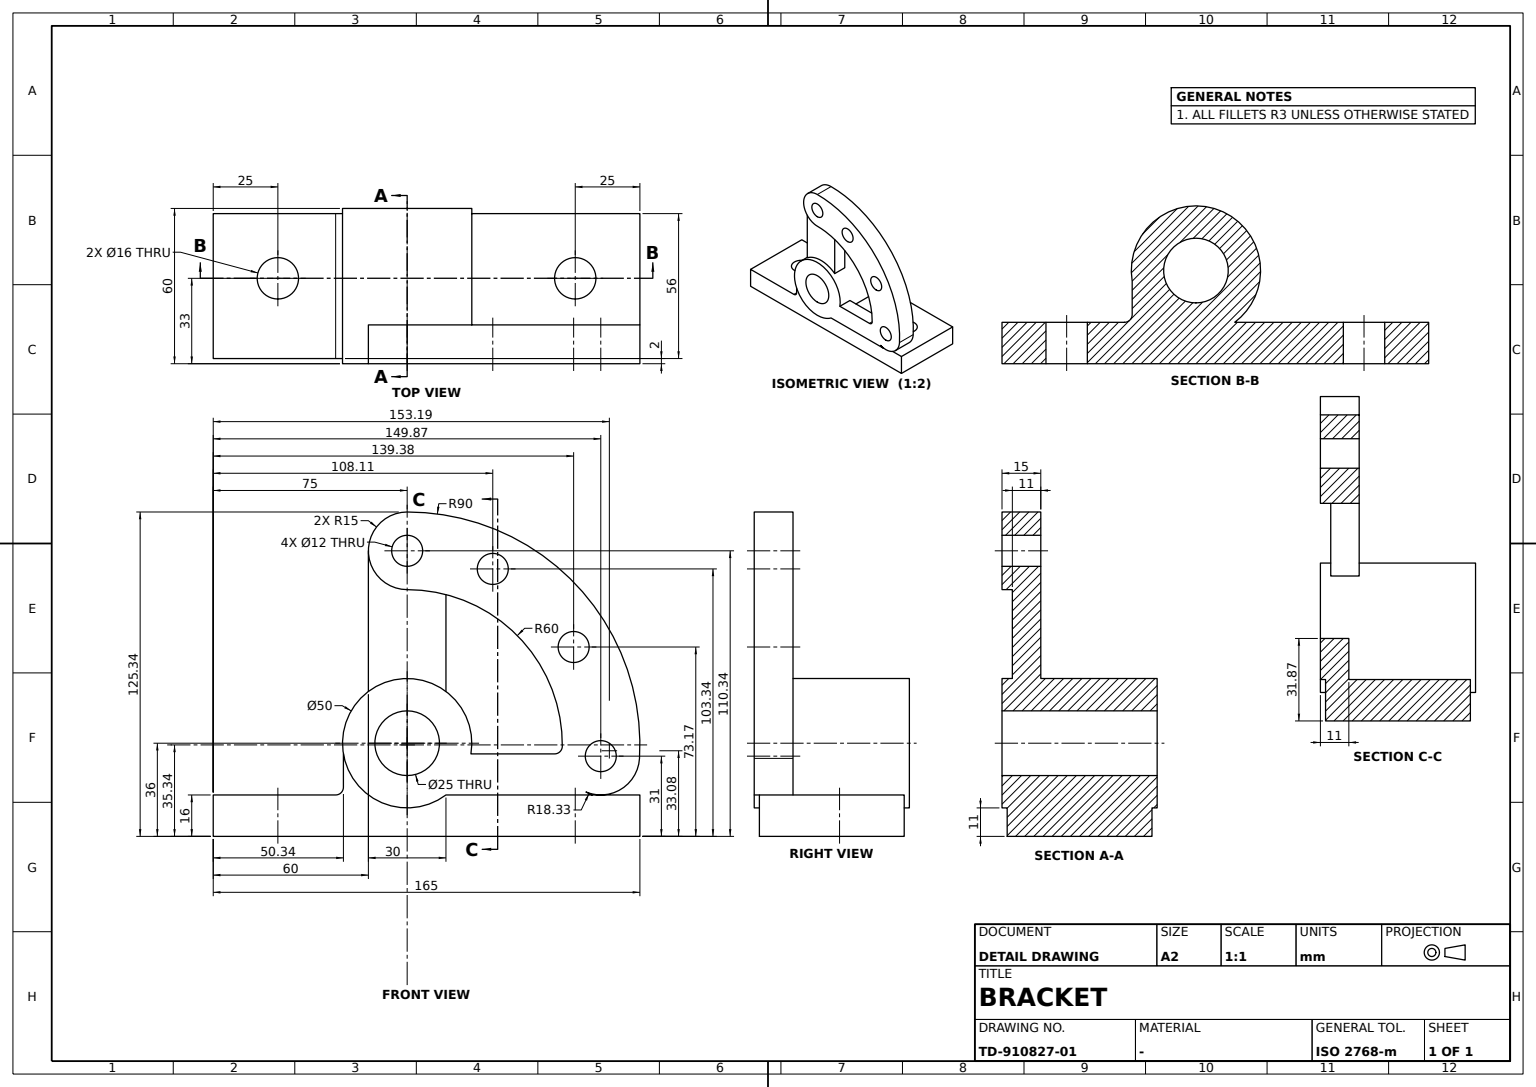
ISO-10303-21;
HEADER;
FILE_DESCRIPTION((''),'2;1');
FILE_NAME('','',(''),(''),'','','');
FILE_SCHEMA(('AUTOMOTIVE_DESIGN'));
ENDSEC;
DATA;
#1=APPLICATION_CONTEXT('');
#2=PRODUCT_CONTEXT('',#1,'mechanical');
#3=PRODUCT('','','',(#2));
#4=PRODUCT_DEFINITION_FORMATION('','',#3);
#5=PRODUCT_DEFINITION_CONTEXT('',#1,'design');
#6=PRODUCT_DEFINITION('','',#4,#5);
#7=PRODUCT_DEFINITION_SHAPE('','',#6);
#8=(LENGTH_UNIT()NAMED_UNIT(*)SI_UNIT(.MILLI.,.METRE.));
#9=(NAMED_UNIT(*)PLANE_ANGLE_UNIT()SI_UNIT($,.RADIAN.));
#10=(NAMED_UNIT(*)SI_UNIT($,.STERADIAN.)SOLID_ANGLE_UNIT());
#11=UNCERTAINTY_MEASURE_WITH_UNIT(LENGTH_MEASURE(0.005),#8,'distance_accuracy_value','');
#12=(GEOMETRIC_REPRESENTATION_CONTEXT(3)GLOBAL_UNCERTAINTY_ASSIGNED_CONTEXT((#11))GLOBAL_UNIT_ASSIGNED_CONTEXT((#8,#9,#10))REPRESENTATION_CONTEXT('',''));
#13=CARTESIAN_POINT('',(15.,0.,104.3383901));
#14=VERTEX_POINT('',#13);
#15=CARTESIAN_POINT('',(15.,0.,110.3383901));
#16=DIRECTION('',(1.,0.,0.));
#17=DIRECTION('',(0.,0.,-1.));
#18=AXIS2_PLACEMENT_3D('',#15,#16,#17);
#19=CIRCLE('',#18,6.);
#20=EDGE_CURVE('',#14,#14,#19,.T.);
#21=ORIENTED_EDGE('',*,*,#20,.T.);
#22=EDGE_LOOP('',(#21));
#23=FACE_BOUND('',#22,.T.);
#24=CARTESIAN_POINT('',(15.,64.37893431,67.16919505));
#25=VERTEX_POINT('',#24);
#26=CARTESIAN_POINT('',(15.,64.37893431,73.16919505));
#27=AXIS2_PLACEMENT_3D('',#26,#16,#17);
#28=CIRCLE('',#27,6.);
#29=EDGE_CURVE('',#25,#25,#28,.T.);
#30=ORIENTED_EDGE('',*,*,#29,.T.);
#31=EDGE_LOOP('',(#30));
#32=FACE_BOUND('',#31,.T.);
#33=CARTESIAN_POINT('',(15.,74.87441734,25.));
#34=VERTEX_POINT('',#33);
#35=CARTESIAN_POINT('',(15.,74.87441734,31.));
#36=AXIS2_PLACEMENT_3D('',#35,#16,#17);
#37=CIRCLE('',#36,6.);
#38=EDGE_CURVE('',#34,#34,#37,.T.);
#39=ORIENTED_EDGE('',*,*,#38,.T.);
#40=EDGE_LOOP('',(#39));
#41=FACE_BOUND('',#40,.T.);
#42=CARTESIAN_POINT('',(15.,33.10708165,97.34314751));
#43=VERTEX_POINT('',#42);
#44=CARTESIAN_POINT('',(15.,33.10708165,103.34314751));
#45=AXIS2_PLACEMENT_3D('',#44,#16,#17);
#46=CIRCLE('',#45,6.);
#47=EDGE_CURVE('',#43,#43,#46,.T.);
#48=ORIENTED_EDGE('',*,*,#47,.T.);
#49=EDGE_LOOP('',(#48));
#50=FACE_BOUND('',#49,.T.);
#51=CARTESIAN_POINT('',(15.,-15.,110.3383901));
#52=VERTEX_POINT('',#51);
#53=CARTESIAN_POINT('',(15.,-15.,56.));
#54=VERTEX_POINT('',#53);
#55=CARTESIAN_POINT('',(15.,-15.,0.));
#56=VECTOR('',#17,1000.);
#57=LINE('',#55,#56);
#58=EDGE_CURVE('',#52,#54,#57,.T.);
#59=ORIENTED_EDGE('',*,*,#58,.F.);
#60=CARTESIAN_POINT('',(15.,0.,125.3383901));
#61=VERTEX_POINT('',#60);
#62=CIRCLE('',#18,15.);
#63=EDGE_CURVE('',#61,#52,#62,.T.);
#64=ORIENTED_EDGE('',*,*,#63,.F.);
#65=CARTESIAN_POINT('',(15.,89.8493008,30.13232198));
#66=VERTEX_POINT('',#65);
#67=CARTESIAN_POINT('',(15.,0.,35.3383901));
#68=AXIS2_PLACEMENT_3D('',#67,#16,#17);
#69=CIRCLE('',#68,90.);
#70=EDGE_CURVE('',#66,#61,#69,.T.);
#71=ORIENTED_EDGE('',*,*,#70,.F.);
#72=CARTESIAN_POINT('',(15.,59.89953387,31.86767802));
#73=VERTEX_POINT('',#72);
#74=CIRCLE('',#36,15.);
#75=EDGE_CURVE('',#73,#66,#74,.T.);
#76=ORIENTED_EDGE('',*,*,#75,.F.);
#77=CARTESIAN_POINT('',(15.,15.,93.4331403));
#78=VERTEX_POINT('',#77);
#79=CIRCLE('',#68,60.);
#80=EDGE_CURVE('',#73,#78,#79,.T.);
#81=ORIENTED_EDGE('',*,*,#80,.T.);
#82=CARTESIAN_POINT('',(15.,15.,56.));
#83=VERTEX_POINT('',#82);
#84=CARTESIAN_POINT('',(15.,15.,0.));
#85=LINE('',#84,#56);
#86=EDGE_CURVE('',#78,#83,#85,.T.);
#87=ORIENTED_EDGE('',*,*,#86,.T.);
#88=CARTESIAN_POINT('',(15.,0.,36.));
#89=AXIS2_PLACEMENT_3D('',#88,#16,#17);
#90=CIRCLE('',#89,25.);
#91=EDGE_CURVE('',#54,#83,#90,.F.);
#92=ORIENTED_EDGE('',*,*,#91,.F.);
#93=EDGE_LOOP('',(#59,#64,#71,#76,#81,#87,#92));
#94=FACE_BOUND('',#93,.T.);
#95=CARTESIAN_POINT('',(15.,0.,0.));
#96=DIRECTION('',(0.,1.,0.));
#97=AXIS2_PLACEMENT_3D('',#95,#16,#96);
#98=PLANE('',#97);
#99=ADVANCED_FACE('',(#23,#32,#41,#50,#94),#98,.F.);
#100=CARTESIAN_POINT('',(28.,-27.65611314,16.));
#101=VERTEX_POINT('',#100);
#102=CARTESIAN_POINT('',(28.,-75.,16.));
#103=VERTEX_POINT('',#102);
#104=CARTESIAN_POINT('',(28.,0.,16.));
#105=DIRECTION('',(0.,-1.,0.));
#106=VECTOR('',#105,1000.);
#107=LINE('',#104,#106);
#108=EDGE_CURVE('',#101,#103,#107,.T.);
#109=ORIENTED_EDGE('',*,*,#108,.T.);
#110=CARTESIAN_POINT('',(28.,-75.,0.));
#111=VERTEX_POINT('',#110);
#112=LINE('',#110,#56);
#113=EDGE_CURVE('',#103,#111,#112,.T.);
#114=ORIENTED_EDGE('',*,*,#113,.T.);
#115=CARTESIAN_POINT('',(28.,90.,0.));
#116=VERTEX_POINT('',#115);
#117=CARTESIAN_POINT('',(28.,0.,0.));
#118=VECTOR('',#96,1000.);
#119=LINE('',#117,#118);
#120=EDGE_CURVE('',#111,#116,#119,.T.);
#121=ORIENTED_EDGE('',*,*,#120,.T.);
#122=CARTESIAN_POINT('',(28.,90.,16.));
#123=VERTEX_POINT('',#122);
#124=DIRECTION('',(0.,0.,1.));
#125=VECTOR('',#124,1000.);
#126=LINE('',#115,#125);
#127=EDGE_CURVE('',#116,#123,#126,.T.);
#128=ORIENTED_EDGE('',*,*,#127,.T.);
#129=CARTESIAN_POINT('',(28.,71.53640747,16.));
#130=VERTEX_POINT('',#129);
#131=EDGE_CURVE('',#123,#130,#107,.T.);
#132=ORIENTED_EDGE('',*,*,#131,.T.);
#133=CARTESIAN_POINT('',(28.,15.,16.));
#134=VERTEX_POINT('',#133);
#135=EDGE_CURVE('',#130,#134,#107,.T.);
#136=ORIENTED_EDGE('',*,*,#135,.T.);
#137=CARTESIAN_POINT('',(28.,-24.65611314,31.86767802));
#138=VERTEX_POINT('',#137);
#139=CARTESIAN_POINT('',(28.,0.,36.));
#140=AXIS2_PLACEMENT_3D('',#139,#16,#17);
#141=CIRCLE('',#140,25.);
#142=EDGE_CURVE('',#138,#134,#141,.T.);
#143=ORIENTED_EDGE('',*,*,#142,.F.);
#144=CARTESIAN_POINT('',(28.,-24.65611314,19.));
#145=VERTEX_POINT('',#144);
#146=LINE('',#137,#56);
#147=EDGE_CURVE('',#138,#145,#146,.T.);
#148=ORIENTED_EDGE('',*,*,#147,.T.);
#149=CARTESIAN_POINT('',(28.,-27.65611314,19.));
#150=AXIS2_PLACEMENT_3D('',#149,#16,#17);
#151=CIRCLE('',#150,3.);
#152=EDGE_CURVE('',#101,#145,#151,.T.);
#153=ORIENTED_EDGE('',*,*,#152,.F.);
#154=EDGE_LOOP('',(#109,#114,#121,#128,#132,#136,#143,#148,#153));
#155=FACE_BOUND('',#154,.T.);
#156=AXIS2_PLACEMENT_3D('',#117,#16,#96);
#157=PLANE('',#156);
#158=ADVANCED_FACE('',(#155),#157,.T.);
#159=CARTESIAN_POINT('',(-11.,-50.,0.));
#160=VERTEX_POINT('',#159);
#161=CARTESIAN_POINT('',(-3.,-50.,0.));
#162=DIRECTION('',(-1.,0.,0.));
#163=AXIS2_PLACEMENT_3D('',#161,#17,#162);
#164=CIRCLE('',#163,8.);
#165=EDGE_CURVE('',#160,#160,#164,.T.);
#166=ORIENTED_EDGE('',*,*,#165,.T.);
#167=EDGE_LOOP('',(#166));
#168=FACE_BOUND('',#167,.T.);
#169=CARTESIAN_POINT('',(5.,-50.,16.));
#170=VERTEX_POINT('',#169);
#171=CARTESIAN_POINT('',(-3.,-50.,16.));
#172=AXIS2_PLACEMENT_3D('',#171,#124,#16);
#173=CIRCLE('',#172,8.);
#174=EDGE_CURVE('',#170,#170,#173,.T.);
#175=ORIENTED_EDGE('',*,*,#174,.T.);
#176=EDGE_LOOP('',(#175));
#177=FACE_BOUND('',#176,.T.);
#178=CARTESIAN_POINT('',(-3.,-50.,7.34));
#179=AXIS2_PLACEMENT_3D('',#178,#124,#16);
#180=CYLINDRICAL_SURFACE('',#179,8.);
#181=ADVANCED_FACE('',(#168,#177),#180,.F.);
#182=CARTESIAN_POINT('',(-28.,-27.65611314,16.));
#183=VERTEX_POINT('',#182);
#184=CARTESIAN_POINT('',(-28.,-75.,16.));
#185=VERTEX_POINT('',#184);
#186=CARTESIAN_POINT('',(-28.,0.,16.));
#187=LINE('',#186,#106);
#188=EDGE_CURVE('',#183,#185,#187,.T.);
#189=ORIENTED_EDGE('',*,*,#188,.F.);
#190=CARTESIAN_POINT('',(-28.,-24.65611314,19.));
#191=VERTEX_POINT('',#190);
#192=CARTESIAN_POINT('',(-28.,-27.65611314,19.));
#193=AXIS2_PLACEMENT_3D('',#192,#16,#17);
#194=CIRCLE('',#193,3.);
#195=EDGE_CURVE('',#183,#191,#194,.T.);
#196=ORIENTED_EDGE('',*,*,#195,.T.);
#197=CARTESIAN_POINT('',(-28.,-24.65611314,31.86767802));
#198=VERTEX_POINT('',#197);
#199=LINE('',#197,#56);
#200=EDGE_CURVE('',#198,#191,#199,.T.);
#201=ORIENTED_EDGE('',*,*,#200,.F.);
#202=CARTESIAN_POINT('',(-28.,15.,16.));
#203=VERTEX_POINT('',#202);
#204=CARTESIAN_POINT('',(-28.,0.,36.));
#205=AXIS2_PLACEMENT_3D('',#204,#16,#17);
#206=CIRCLE('',#205,25.);
#207=EDGE_CURVE('',#198,#203,#206,.T.);
#208=ORIENTED_EDGE('',*,*,#207,.T.);
#209=CARTESIAN_POINT('',(-28.,90.,16.));
#210=VERTEX_POINT('',#209);
#211=EDGE_CURVE('',#210,#203,#187,.T.);
#212=ORIENTED_EDGE('',*,*,#211,.F.);
#213=CARTESIAN_POINT('',(-28.,90.,0.));
#214=VERTEX_POINT('',#213);
#215=LINE('',#213,#125);
#216=EDGE_CURVE('',#214,#210,#215,.T.);
#217=ORIENTED_EDGE('',*,*,#216,.F.);
#218=CARTESIAN_POINT('',(-28.,-75.,0.));
#219=VERTEX_POINT('',#218);
#220=CARTESIAN_POINT('',(-28.,0.,0.));
#221=LINE('',#220,#118);
#222=EDGE_CURVE('',#219,#214,#221,.T.);
#223=ORIENTED_EDGE('',*,*,#222,.F.);
#224=LINE('',#218,#56);
#225=EDGE_CURVE('',#185,#219,#224,.T.);
#226=ORIENTED_EDGE('',*,*,#225,.F.);
#227=EDGE_LOOP('',(#189,#196,#201,#208,#212,#217,#223,#226));
#228=FACE_BOUND('',#227,.T.);
#229=AXIS2_PLACEMENT_3D('',#220,#16,#96);
#230=PLANE('',#229);
#231=ADVANCED_FACE('',(#228),#230,.F.);
#232=ORIENTED_EDGE('',*,*,#200,.T.);
#233=CARTESIAN_POINT('',(0.,-24.65611314,19.));
#234=VECTOR('',#16,1000.);
#235=LINE('',#233,#234);
#236=EDGE_CURVE('',#191,#145,#235,.T.);
#237=ORIENTED_EDGE('',*,*,#236,.T.);
#238=ORIENTED_EDGE('',*,*,#147,.F.);
#239=LINE('',#137,#234);
#240=EDGE_CURVE('',#138,#198,#239,.F.);
#241=ORIENTED_EDGE('',*,*,#240,.T.);
#242=EDGE_LOOP('',(#232,#237,#238,#241));
#243=FACE_BOUND('',#242,.T.);
#244=AXIS2_PLACEMENT_3D('',#137,#96,#17);
#245=PLANE('',#244);
#246=ADVANCED_FACE('',(#243),#245,.F.);
#247=CARTESIAN_POINT('',(30.,33.10708165,97.34314751));
#248=VERTEX_POINT('',#247);
#249=CARTESIAN_POINT('',(30.,33.10708165,103.34314751));
#250=AXIS2_PLACEMENT_3D('',#249,#16,#17);
#251=CIRCLE('',#250,6.);
#252=EDGE_CURVE('',#248,#248,#251,.T.);
#253=ORIENTED_EDGE('',*,*,#252,.T.);
#254=EDGE_LOOP('',(#253));
#255=FACE_BOUND('',#254,.T.);
#256=ORIENTED_EDGE('',*,*,#47,.F.);
#257=EDGE_LOOP('',(#256));
#258=FACE_BOUND('',#257,.T.);
#259=CARTESIAN_POINT('',(-0.66,33.10708165,103.34314751));
#260=AXIS2_PLACEMENT_3D('',#259,#16,#96);
#261=CYLINDRICAL_SURFACE('',#260,6.);
#262=ADVANCED_FACE('',(#255,#258),#261,.F.);
#263=CARTESIAN_POINT('',(30.,0.,104.3383901));
#264=VERTEX_POINT('',#263);
#265=CARTESIAN_POINT('',(30.,0.,110.3383901));
#266=AXIS2_PLACEMENT_3D('',#265,#16,#17);
#267=CIRCLE('',#266,6.);
#268=EDGE_CURVE('',#264,#264,#267,.T.);
#269=ORIENTED_EDGE('',*,*,#268,.T.);
#270=EDGE_LOOP('',(#269));
#271=FACE_BOUND('',#270,.T.);
#272=ORIENTED_EDGE('',*,*,#20,.F.);
#273=EDGE_LOOP('',(#272));
#274=FACE_BOUND('',#273,.T.);
#275=CARTESIAN_POINT('',(-0.66,0.,110.3383901));
#276=AXIS2_PLACEMENT_3D('',#275,#16,#96);
#277=CYLINDRICAL_SURFACE('',#276,6.);
#278=ADVANCED_FACE('',(#271,#274),#277,.F.);
#279=ORIENTED_EDGE('',*,*,#252,.F.);
#280=EDGE_LOOP('',(#279));
#281=FACE_BOUND('',#280,.T.);
#282=CARTESIAN_POINT('',(30.,24.65611314,31.86767802));
#283=VERTEX_POINT('',#282);
#284=CARTESIAN_POINT('',(30.,15.,16.));
#285=VERTEX_POINT('',#284);
#286=CARTESIAN_POINT('',(30.,0.,36.));
#287=AXIS2_PLACEMENT_3D('',#286,#16,#17);
#288=CIRCLE('',#287,25.);
#289=EDGE_CURVE('',#283,#285,#288,.T.);
#290=ORIENTED_EDGE('',*,*,#289,.T.);
#291=CARTESIAN_POINT('',(30.,71.53640747,16.));
#292=VERTEX_POINT('',#291);
#293=CARTESIAN_POINT('',(30.,90.,16.));
#294=LINE('',#293,#118);
#295=EDGE_CURVE('',#285,#292,#294,.T.);
#296=ORIENTED_EDGE('',*,*,#295,.T.);
#297=CARTESIAN_POINT('',(30.,69.14079351,17.1390636));
#298=VERTEX_POINT('',#297);
#299=CARTESIAN_POINT('',(30.,78.18875671,33.07953511));
#300=AXIS2_PLACEMENT_3D('',#299,#16,#17);
#301=CIRCLE('',#300,18.32932814);
#302=EDGE_CURVE('',#298,#292,#301,.T.);
#303=ORIENTED_EDGE('',*,*,#302,.F.);
#304=CARTESIAN_POINT('',(30.,89.8493008,30.13232198));
#305=VERTEX_POINT('',#304);
#306=CARTESIAN_POINT('',(30.,74.87441734,31.));
#307=AXIS2_PLACEMENT_3D('',#306,#16,#17);
#308=CIRCLE('',#307,15.);
#309=EDGE_CURVE('',#298,#305,#308,.T.);
#310=ORIENTED_EDGE('',*,*,#309,.T.);
#311=CARTESIAN_POINT('',(30.,0.,125.3383901));
#312=VERTEX_POINT('',#311);
#313=CARTESIAN_POINT('',(30.,0.,35.3383901));
#314=AXIS2_PLACEMENT_3D('',#313,#16,#17);
#315=CIRCLE('',#314,90.);
#316=EDGE_CURVE('',#305,#312,#315,.T.);
#317=ORIENTED_EDGE('',*,*,#316,.T.);
#318=CARTESIAN_POINT('',(30.,0.,95.3383901));
#319=VERTEX_POINT('',#318);
#320=CIRCLE('',#266,15.);
#321=EDGE_CURVE('',#312,#319,#320,.T.);
#322=ORIENTED_EDGE('',*,*,#321,.T.);
#323=CARTESIAN_POINT('',(30.,59.99795408,34.8429037));
#324=VERTEX_POINT('',#323);
#325=CIRCLE('',#314,60.);
#326=EDGE_CURVE('',#324,#319,#325,.T.);
#327=ORIENTED_EDGE('',*,*,#326,.F.);
#328=CARTESIAN_POINT('',(30.,56.99805637,31.86767802));
#329=VERTEX_POINT('',#328);
#330=CARTESIAN_POINT('',(30.,56.99805637,34.86767802));
#331=AXIS2_PLACEMENT_3D('',#330,#16,#17);
#332=CIRCLE('',#331,3.);
#333=EDGE_CURVE('',#329,#324,#332,.T.);
#334=ORIENTED_EDGE('',*,*,#333,.F.);
#335=CARTESIAN_POINT('',(30.,59.89953387,31.86767802));
#336=LINE('',#335,#106);
#337=EDGE_CURVE('',#329,#283,#336,.T.);
#338=ORIENTED_EDGE('',*,*,#337,.T.);
#339=EDGE_LOOP('',(#290,#296,#303,#310,#317,#322,#327,#334,#338));
#340=FACE_BOUND('',#339,.T.);
#341=CARTESIAN_POINT('',(30.,74.87441734,25.));
#342=VERTEX_POINT('',#341);
#343=CIRCLE('',#307,6.);
#344=EDGE_CURVE('',#342,#342,#343,.T.);
#345=ORIENTED_EDGE('',*,*,#344,.F.);
#346=EDGE_LOOP('',(#345));
#347=FACE_BOUND('',#346,.T.);
#348=CARTESIAN_POINT('',(30.,64.37893431,67.16919505));
#349=VERTEX_POINT('',#348);
#350=CARTESIAN_POINT('',(30.,64.37893431,73.16919505));
#351=AXIS2_PLACEMENT_3D('',#350,#16,#17);
#352=CIRCLE('',#351,6.);
#353=EDGE_CURVE('',#349,#349,#352,.T.);
#354=ORIENTED_EDGE('',*,*,#353,.F.);
#355=EDGE_LOOP('',(#354));
#356=FACE_BOUND('',#355,.T.);
#357=CARTESIAN_POINT('',(30.,0.,23.5));
#358=VERTEX_POINT('',#357);
#359=CIRCLE('',#287,12.5);
#360=EDGE_CURVE('',#358,#358,#359,.T.);
#361=ORIENTED_EDGE('',*,*,#360,.F.);
#362=EDGE_LOOP('',(#361));
#363=FACE_BOUND('',#362,.T.);
#364=ORIENTED_EDGE('',*,*,#268,.F.);
#365=EDGE_LOOP('',(#364));
#366=FACE_BOUND('',#365,.T.);
#367=CARTESIAN_POINT('',(30.,0.,0.));
#368=AXIS2_PLACEMENT_3D('',#367,#16,#96);
#369=PLANE('',#368);
#370=ADVANCED_FACE('',(#281,#340,#347,#356,#363,#366),#369,.T.);
#371=ORIENTED_EDGE('',*,*,#360,.T.);
#372=EDGE_LOOP('',(#371));
#373=FACE_BOUND('',#372,.T.);
#374=CARTESIAN_POINT('',(-30.,0.,23.5));
#375=VERTEX_POINT('',#374);
#376=CARTESIAN_POINT('',(-30.,0.,36.));
#377=AXIS2_PLACEMENT_3D('',#376,#16,#17);
#378=CIRCLE('',#377,12.5);
#379=EDGE_CURVE('',#375,#375,#378,.T.);
#380=ORIENTED_EDGE('',*,*,#379,.F.);
#381=EDGE_LOOP('',(#380));
#382=FACE_BOUND('',#381,.T.);
#383=CARTESIAN_POINT('',(0.,0.,36.));
#384=AXIS2_PLACEMENT_3D('',#383,#16,#96);
#385=CYLINDRICAL_SURFACE('',#384,12.5);
#386=ADVANCED_FACE('',(#373,#382),#385,.F.);
#387=CARTESIAN_POINT('',(19.,56.99805637,31.86767802));
#388=VERTEX_POINT('',#387);
#389=CARTESIAN_POINT('',(19.,24.65611314,31.86767802));
#390=VERTEX_POINT('',#389);
#391=CARTESIAN_POINT('',(19.,59.89953387,31.86767802));
#392=LINE('',#391,#106);
#393=EDGE_CURVE('',#388,#390,#392,.T.);
#394=ORIENTED_EDGE('',*,*,#393,.T.);
#395=LINE('',#282,#234);
#396=EDGE_CURVE('',#283,#390,#395,.F.);
#397=ORIENTED_EDGE('',*,*,#396,.F.);
#398=ORIENTED_EDGE('',*,*,#337,.F.);
#399=CARTESIAN_POINT('',(22.5,56.99805637,31.86767802));
#400=VECTOR('',#162,1000.);
#401=LINE('',#399,#400);
#402=EDGE_CURVE('',#329,#388,#401,.T.);
#403=ORIENTED_EDGE('',*,*,#402,.T.);
#404=EDGE_LOOP('',(#394,#397,#398,#403));
#405=FACE_BOUND('',#404,.T.);
#406=AXIS2_PLACEMENT_3D('',#335,#17,#105);
#407=PLANE('',#406);
#408=ADVANCED_FACE('',(#405),#407,.F.);
#409=ORIENTED_EDGE('',*,*,#174,.F.);
#410=EDGE_LOOP('',(#409));
#411=FACE_BOUND('',#410,.T.);
#412=ORIENTED_EDGE('',*,*,#188,.T.);
#413=CARTESIAN_POINT('',(0.,-75.,16.));
#414=LINE('',#413,#234);
#415=EDGE_CURVE('',#185,#103,#414,.T.);
#416=ORIENTED_EDGE('',*,*,#415,.T.);
#417=ORIENTED_EDGE('',*,*,#108,.F.);
#418=CARTESIAN_POINT('',(0.,-27.65611314,16.));
#419=LINE('',#418,#234);
#420=EDGE_CURVE('',#183,#101,#419,.T.);
#421=ORIENTED_EDGE('',*,*,#420,.F.);
#422=EDGE_LOOP('',(#412,#416,#417,#421));
#423=FACE_BOUND('',#422,.T.);
#424=CARTESIAN_POINT('',(0.,90.,16.));
#425=AXIS2_PLACEMENT_3D('',#424,#124,#105);
#426=PLANE('',#425);
#427=ADVANCED_FACE('',(#411,#423),#426,.T.);
#428=CARTESIAN_POINT('',(26.,-15.,56.));
#429=VERTEX_POINT('',#428);
#430=LINE('',#53,#234);
#431=EDGE_CURVE('',#54,#429,#430,.T.);
#432=ORIENTED_EDGE('',*,*,#431,.T.);
#433=CARTESIAN_POINT('',(26.,-15.,110.3383901));
#434=VERTEX_POINT('',#433);
#435=LINE('',#433,#56);
#436=EDGE_CURVE('',#434,#429,#435,.T.);
#437=ORIENTED_EDGE('',*,*,#436,.F.);
#438=CARTESIAN_POINT('',(22.5,-15.,110.3383901));
#439=LINE('',#438,#234);
#440=EDGE_CURVE('',#52,#434,#439,.T.);
#441=ORIENTED_EDGE('',*,*,#440,.F.);
#442=ORIENTED_EDGE('',*,*,#58,.T.);
#443=EDGE_LOOP('',(#432,#437,#441,#442));
#444=FACE_BOUND('',#443,.T.);
#445=AXIS2_PLACEMENT_3D('',#51,#105,#17);
#446=PLANE('',#445);
#447=ADVANCED_FACE('',(#444),#446,.T.);
#448=CARTESIAN_POINT('',(26.,15.,56.));
#449=VERTEX_POINT('',#448);
#450=LINE('',#82,#234);
#451=EDGE_CURVE('',#83,#449,#450,.T.);
#452=ORIENTED_EDGE('',*,*,#451,.T.);
#453=CARTESIAN_POINT('',(26.,0.,36.));
#454=AXIS2_PLACEMENT_3D('',#453,#162,#124);
#455=CIRCLE('',#454,25.);
#456=EDGE_CURVE('',#429,#449,#455,.T.);
#457=ORIENTED_EDGE('',*,*,#456,.F.);
#458=ORIENTED_EDGE('',*,*,#431,.F.);
#459=ORIENTED_EDGE('',*,*,#91,.T.);
#460=EDGE_LOOP('',(#452,#457,#458,#459));
#461=FACE_BOUND('',#460,.T.);
#462=ORIENTED_EDGE('',*,*,#142,.T.);
#463=LINE('',#284,#234);
#464=EDGE_CURVE('',#285,#134,#463,.F.);
#465=ORIENTED_EDGE('',*,*,#464,.F.);
#466=ORIENTED_EDGE('',*,*,#289,.F.);
#467=ORIENTED_EDGE('',*,*,#396,.T.);
#468=CARTESIAN_POINT('',(19.,15.,16.));
#469=VERTEX_POINT('',#468);
#470=CARTESIAN_POINT('',(19.,0.,36.));
#471=AXIS2_PLACEMENT_3D('',#470,#16,#17);
#472=CIRCLE('',#471,25.);
#473=EDGE_CURVE('',#469,#390,#472,.T.);
#474=ORIENTED_EDGE('',*,*,#473,.F.);
#475=LINE('',#202,#234);
#476=EDGE_CURVE('',#203,#469,#475,.T.);
#477=ORIENTED_EDGE('',*,*,#476,.F.);
#478=ORIENTED_EDGE('',*,*,#207,.F.);
#479=ORIENTED_EDGE('',*,*,#240,.F.);
#480=EDGE_LOOP('',(#462,#465,#466,#467,#474,#477,#478,#479));
#481=FACE_BOUND('',#480,.T.);
#482=CARTESIAN_POINT('',(-30.,0.,11.));
#483=VERTEX_POINT('',#482);
#484=CIRCLE('',#377,25.);
#485=EDGE_CURVE('',#483,#483,#484,.T.);
#486=ORIENTED_EDGE('',*,*,#485,.T.);
#487=EDGE_LOOP('',(#486));
#488=FACE_BOUND('',#487,.T.);
#489=CYLINDRICAL_SURFACE('',#384,25.);
#490=ADVANCED_FACE('',(#461,#481,#488),#489,.T.);
#491=CARTESIAN_POINT('',(26.,0.,95.3383901));
#492=VERTEX_POINT('',#491);
#493=CARTESIAN_POINT('',(28.,0.,95.3383901));
#494=LINE('',#493,#234);
#495=EDGE_CURVE('',#319,#492,#494,.F.);
#496=ORIENTED_EDGE('',*,*,#495,.F.);
#497=ORIENTED_EDGE('',*,*,#321,.F.);
#498=CARTESIAN_POINT('',(22.5,0.,125.3383901));
#499=LINE('',#498,#234);
#500=EDGE_CURVE('',#312,#61,#499,.F.);
#501=ORIENTED_EDGE('',*,*,#500,.T.);
#502=ORIENTED_EDGE('',*,*,#63,.T.);
#503=ORIENTED_EDGE('',*,*,#440,.T.);
#504=CARTESIAN_POINT('',(26.,0.,110.3383901));
#505=AXIS2_PLACEMENT_3D('',#504,#162,#124);
#506=CIRCLE('',#505,15.);
#507=EDGE_CURVE('',#492,#434,#506,.T.);
#508=ORIENTED_EDGE('',*,*,#507,.F.);
#509=EDGE_LOOP('',(#496,#497,#501,#502,#503,#508));
#510=FACE_BOUND('',#509,.T.);
#511=CARTESIAN_POINT('',(22.5,0.,110.3383901));
#512=AXIS2_PLACEMENT_3D('',#511,#16,#96);
#513=CYLINDRICAL_SURFACE('',#512,15.);
#514=ADVANCED_FACE('',(#510),#513,.T.);
#515=CARTESIAN_POINT('',(19.,69.14079351,17.1390636));
#516=VERTEX_POINT('',#515);
#517=LINE('',#297,#234);
#518=EDGE_CURVE('',#298,#516,#517,.F.);
#519=ORIENTED_EDGE('',*,*,#518,.T.);
#520=VERTEX_POINT('',#391);
#521=CARTESIAN_POINT('',(19.,74.87441734,31.));
#522=AXIS2_PLACEMENT_3D('',#521,#16,#17);
#523=CIRCLE('',#522,15.);
#524=EDGE_CURVE('',#520,#516,#523,.T.);
#525=ORIENTED_EDGE('',*,*,#524,.F.);
#526=CARTESIAN_POINT('',(17.,59.89953387,31.86767802));
#527=LINE('',#526,#234);
#528=EDGE_CURVE('',#520,#73,#527,.F.);
#529=ORIENTED_EDGE('',*,*,#528,.T.);
#530=ORIENTED_EDGE('',*,*,#75,.T.);
#531=CARTESIAN_POINT('',(22.5,89.8493008,30.13232198));
#532=LINE('',#531,#234);
#533=EDGE_CURVE('',#305,#66,#532,.F.);
#534=ORIENTED_EDGE('',*,*,#533,.F.);
#535=ORIENTED_EDGE('',*,*,#309,.F.);
#536=EDGE_LOOP('',(#519,#525,#529,#530,#534,#535));
#537=FACE_BOUND('',#536,.T.);
#538=CARTESIAN_POINT('',(22.5,74.87441734,31.));
#539=AXIS2_PLACEMENT_3D('',#538,#16,#96);
#540=CYLINDRICAL_SURFACE('',#539,15.);
#541=ADVANCED_FACE('',(#537),#540,.T.);
#542=CARTESIAN_POINT('',(0.,-75.,0.));
#543=LINE('',#542,#234);
#544=EDGE_CURVE('',#219,#111,#543,.T.);
#545=ORIENTED_EDGE('',*,*,#544,.T.);
#546=ORIENTED_EDGE('',*,*,#113,.F.);
#547=ORIENTED_EDGE('',*,*,#415,.F.);
#548=ORIENTED_EDGE('',*,*,#225,.T.);
#549=EDGE_LOOP('',(#545,#546,#547,#548));
#550=FACE_BOUND('',#549,.T.);
#551=AXIS2_PLACEMENT_3D('',#413,#105,#17);
#552=PLANE('',#551);
#553=ADVANCED_FACE('',(#550),#552,.T.);
#554=ORIENTED_EDGE('',*,*,#544,.F.);
#555=ORIENTED_EDGE('',*,*,#222,.T.);
#556=CARTESIAN_POINT('',(0.,90.,0.));
#557=LINE('',#556,#234);
#558=EDGE_CURVE('',#214,#116,#557,.T.);
#559=ORIENTED_EDGE('',*,*,#558,.T.);
#560=ORIENTED_EDGE('',*,*,#120,.F.);
#561=EDGE_LOOP('',(#554,#555,#559,#560));
#562=FACE_BOUND('',#561,.T.);
#563=ORIENTED_EDGE('',*,*,#165,.F.);
#564=EDGE_LOOP('',(#563));
#565=FACE_BOUND('',#564,.T.);
#566=CARTESIAN_POINT('',(-11.,65.,0.));
#567=VERTEX_POINT('',#566);
#568=CARTESIAN_POINT('',(-3.,65.,0.));
#569=AXIS2_PLACEMENT_3D('',#568,#17,#162);
#570=CIRCLE('',#569,8.);
#571=EDGE_CURVE('',#567,#567,#570,.T.);
#572=ORIENTED_EDGE('',*,*,#571,.F.);
#573=EDGE_LOOP('',(#572));
#574=FACE_BOUND('',#573,.T.);
#575=AXIS2_PLACEMENT_3D('',#542,#17,#96);
#576=PLANE('',#575);
#577=ADVANCED_FACE('',(#562,#565,#574),#576,.T.);
#578=ORIENTED_EDGE('',*,*,#38,.F.);
#579=EDGE_LOOP('',(#578));
#580=FACE_BOUND('',#579,.T.);
#581=ORIENTED_EDGE('',*,*,#344,.T.);
#582=EDGE_LOOP('',(#581));
#583=FACE_BOUND('',#582,.T.);
#584=CARTESIAN_POINT('',(-0.66,74.87441734,31.));
#585=AXIS2_PLACEMENT_3D('',#584,#16,#96);
#586=CYLINDRICAL_SURFACE('',#585,6.);
#587=ADVANCED_FACE('',(#580,#583),#586,.F.);
#588=LINE('',#424,#234);
#589=EDGE_CURVE('',#210,#123,#588,.T.);
#590=ORIENTED_EDGE('',*,*,#589,.F.);
#591=ORIENTED_EDGE('',*,*,#211,.T.);
#592=ORIENTED_EDGE('',*,*,#476,.T.);
#593=CARTESIAN_POINT('',(19.,71.53640747,16.));
#594=VERTEX_POINT('',#593);
#595=CARTESIAN_POINT('',(19.,90.,16.));
#596=LINE('',#595,#118);
#597=EDGE_CURVE('',#469,#594,#596,.T.);
#598=ORIENTED_EDGE('',*,*,#597,.T.);
#599=LINE('',#129,#234);
#600=EDGE_CURVE('',#130,#594,#599,.F.);
#601=ORIENTED_EDGE('',*,*,#600,.F.);
#602=ORIENTED_EDGE('',*,*,#131,.F.);
#603=EDGE_LOOP('',(#590,#591,#592,#598,#601,#602));
#604=FACE_BOUND('',#603,.T.);
#605=CARTESIAN_POINT('',(5.,65.,16.));
#606=VERTEX_POINT('',#605);
#607=CARTESIAN_POINT('',(-3.,65.,16.));
#608=AXIS2_PLACEMENT_3D('',#607,#124,#16);
#609=CIRCLE('',#608,8.);
#610=EDGE_CURVE('',#606,#606,#609,.T.);
#611=ORIENTED_EDGE('',*,*,#610,.F.);
#612=EDGE_LOOP('',(#611));
#613=FACE_BOUND('',#612,.T.);
#614=ADVANCED_FACE('',(#604,#613),#426,.T.);
#615=ORIENTED_EDGE('',*,*,#302,.T.);
#616=LINE('',#291,#234);
#617=EDGE_CURVE('',#292,#130,#616,.F.);
#618=ORIENTED_EDGE('',*,*,#617,.T.);
#619=ORIENTED_EDGE('',*,*,#600,.T.);
#620=CARTESIAN_POINT('',(19.,78.18875671,33.07953511));
#621=AXIS2_PLACEMENT_3D('',#620,#16,#17);
#622=CIRCLE('',#621,18.32932814);
#623=EDGE_CURVE('',#516,#594,#622,.T.);
#624=ORIENTED_EDGE('',*,*,#623,.F.);
#625=ORIENTED_EDGE('',*,*,#518,.F.);
#626=EDGE_LOOP('',(#615,#618,#619,#624,#625));
#627=FACE_BOUND('',#626,.T.);
#628=CARTESIAN_POINT('',(24.5,78.18875671,33.07953511));
#629=AXIS2_PLACEMENT_3D('',#628,#16,#96);
#630=CYLINDRICAL_SURFACE('',#629,18.32932814);
#631=ADVANCED_FACE('',(#627),#630,.F.);
#632=ORIENTED_EDGE('',*,*,#617,.F.);
#633=ORIENTED_EDGE('',*,*,#295,.F.);
#634=ORIENTED_EDGE('',*,*,#464,.T.);
#635=ORIENTED_EDGE('',*,*,#135,.F.);
#636=EDGE_LOOP('',(#632,#633,#634,#635));
#637=FACE_BOUND('',#636,.T.);
#638=ADVANCED_FACE('',(#637),#426,.F.);
#639=ORIENTED_EDGE('',*,*,#533,.T.);
#640=ORIENTED_EDGE('',*,*,#70,.T.);
#641=ORIENTED_EDGE('',*,*,#500,.F.);
#642=ORIENTED_EDGE('',*,*,#316,.F.);
#643=EDGE_LOOP('',(#639,#640,#641,#642));
#644=FACE_BOUND('',#643,.T.);
#645=CARTESIAN_POINT('',(22.5,0.,35.3383901));
#646=AXIS2_PLACEMENT_3D('',#645,#16,#96);
#647=CYLINDRICAL_SURFACE('',#646,90.);
#648=ADVANCED_FACE('',(#644),#647,.T.);
#649=ORIENTED_EDGE('',*,*,#379,.T.);
#650=EDGE_LOOP('',(#649));
#651=FACE_BOUND('',#650,.T.);
#652=ORIENTED_EDGE('',*,*,#485,.F.);
#653=EDGE_LOOP('',(#652));
#654=FACE_BOUND('',#653,.T.);
#655=CARTESIAN_POINT('',(-30.,0.,0.));
#656=AXIS2_PLACEMENT_3D('',#655,#16,#96);
#657=PLANE('',#656);
#658=ADVANCED_FACE('',(#651,#654),#657,.F.);
#659=ORIENTED_EDGE('',*,*,#623,.T.);
#660=ORIENTED_EDGE('',*,*,#597,.F.);
#661=ORIENTED_EDGE('',*,*,#473,.T.);
#662=ORIENTED_EDGE('',*,*,#393,.F.);
#663=CARTESIAN_POINT('',(19.,59.99795408,34.8429037));
#664=VERTEX_POINT('',#663);
#665=CARTESIAN_POINT('',(19.,56.99805637,34.86767802));
#666=AXIS2_PLACEMENT_3D('',#665,#16,#17);
#667=CIRCLE('',#666,3.);
#668=EDGE_CURVE('',#388,#664,#667,.T.);
#669=ORIENTED_EDGE('',*,*,#668,.T.);
#670=CARTESIAN_POINT('',(19.,0.,35.3383901));
#671=AXIS2_PLACEMENT_3D('',#670,#16,#17);
#672=CIRCLE('',#671,60.);
#673=EDGE_CURVE('',#520,#664,#672,.T.);
#674=ORIENTED_EDGE('',*,*,#673,.F.);
#675=ORIENTED_EDGE('',*,*,#524,.T.);
#676=EDGE_LOOP('',(#659,#660,#661,#662,#669,#674,#675));
#677=FACE_BOUND('',#676,.T.);
#678=CARTESIAN_POINT('',(19.,0.,0.));
#679=AXIS2_PLACEMENT_3D('',#678,#16,#96);
#680=PLANE('',#679);
#681=ADVANCED_FACE('',(#677),#680,.F.);
#682=ORIENTED_EDGE('',*,*,#353,.T.);
#683=EDGE_LOOP('',(#682));
#684=FACE_BOUND('',#683,.T.);
#685=ORIENTED_EDGE('',*,*,#29,.F.);
#686=EDGE_LOOP('',(#685));
#687=FACE_BOUND('',#686,.T.);
#688=CARTESIAN_POINT('',(-0.66,64.37893431,73.16919505));
#689=AXIS2_PLACEMENT_3D('',#688,#16,#96);
#690=CYLINDRICAL_SURFACE('',#689,6.);
#691=ADVANCED_FACE('',(#684,#687),#690,.F.);
#692=CARTESIAN_POINT('',(24.5,59.99795408,34.8429037));
#693=LINE('',#692,#234);
#694=EDGE_CURVE('',#324,#664,#693,.F.);
#695=ORIENTED_EDGE('',*,*,#694,.F.);
#696=ORIENTED_EDGE('',*,*,#326,.T.);
#697=ORIENTED_EDGE('',*,*,#495,.T.);
#698=CARTESIAN_POINT('',(26.,15.,93.4331403));
#699=VERTEX_POINT('',#698);
#700=CARTESIAN_POINT('',(26.,0.,35.3383901));
#701=AXIS2_PLACEMENT_3D('',#700,#162,#124);
#702=CIRCLE('',#701,60.);
#703=EDGE_CURVE('',#492,#699,#702,.T.);
#704=ORIENTED_EDGE('',*,*,#703,.T.);
#705=LINE('',#77,#234);
#706=EDGE_CURVE('',#78,#699,#705,.T.);
#707=ORIENTED_EDGE('',*,*,#706,.F.);
#708=ORIENTED_EDGE('',*,*,#80,.F.);
#709=ORIENTED_EDGE('',*,*,#528,.F.);
#710=ORIENTED_EDGE('',*,*,#673,.T.);
#711=EDGE_LOOP('',(#695,#696,#697,#704,#707,#708,#709,#710));
#712=FACE_BOUND('',#711,.T.);
#713=CYLINDRICAL_SURFACE('',#646,60.);
#714=ADVANCED_FACE('',(#712),#713,.F.);
#715=ORIENTED_EDGE('',*,*,#706,.T.);
#716=LINE('',#698,#56);
#717=EDGE_CURVE('',#699,#449,#716,.T.);
#718=ORIENTED_EDGE('',*,*,#717,.T.);
#719=ORIENTED_EDGE('',*,*,#451,.F.);
#720=ORIENTED_EDGE('',*,*,#86,.F.);
#721=EDGE_LOOP('',(#715,#718,#719,#720));
#722=FACE_BOUND('',#721,.T.);
#723=AXIS2_PLACEMENT_3D('',#77,#105,#17);
#724=PLANE('',#723);
#725=ADVANCED_FACE('',(#722),#724,.F.);
#726=ORIENTED_EDGE('',*,*,#195,.F.);
#727=ORIENTED_EDGE('',*,*,#420,.T.);
#728=ORIENTED_EDGE('',*,*,#152,.T.);
#729=ORIENTED_EDGE('',*,*,#236,.F.);
#730=EDGE_LOOP('',(#726,#727,#728,#729));
#731=FACE_BOUND('',#730,.T.);
#732=CARTESIAN_POINT('',(0.,-27.65611314,19.));
#733=AXIS2_PLACEMENT_3D('',#732,#16,#96);
#734=CYLINDRICAL_SURFACE('',#733,3.);
#735=ADVANCED_FACE('',(#731),#734,.F.);
#736=ORIENTED_EDGE('',*,*,#694,.T.);
#737=ORIENTED_EDGE('',*,*,#668,.F.);
#738=ORIENTED_EDGE('',*,*,#402,.F.);
#739=ORIENTED_EDGE('',*,*,#333,.T.);
#740=EDGE_LOOP('',(#736,#737,#738,#739));
#741=FACE_BOUND('',#740,.T.);
#742=CARTESIAN_POINT('',(22.5,56.99805637,34.86767802));
#743=DIRECTION('',(0.,0.999965901,-0.008258107));
#744=AXIS2_PLACEMENT_3D('',#742,#162,#743);
#745=CYLINDRICAL_SURFACE('',#744,3.);
#746=ADVANCED_FACE('',(#741),#745,.F.);
#747=ORIENTED_EDGE('',*,*,#610,.T.);
#748=EDGE_LOOP('',(#747));
#749=FACE_BOUND('',#748,.T.);
#750=ORIENTED_EDGE('',*,*,#571,.T.);
#751=EDGE_LOOP('',(#750));
#752=FACE_BOUND('',#751,.T.);
#753=CARTESIAN_POINT('',(-3.,65.,7.34));
#754=AXIS2_PLACEMENT_3D('',#753,#124,#16);
#755=CYLINDRICAL_SURFACE('',#754,8.);
#756=ADVANCED_FACE('',(#749,#752),#755,.F.);
#757=ORIENTED_EDGE('',*,*,#558,.F.);
#758=ORIENTED_EDGE('',*,*,#216,.T.);
#759=ORIENTED_EDGE('',*,*,#589,.T.);
#760=ORIENTED_EDGE('',*,*,#127,.F.);
#761=EDGE_LOOP('',(#757,#758,#759,#760));
#762=FACE_BOUND('',#761,.T.);
#763=AXIS2_PLACEMENT_3D('',#556,#96,#124);
#764=PLANE('',#763);
#765=ADVANCED_FACE('',(#762),#764,.T.);
#766=ORIENTED_EDGE('',*,*,#703,.F.);
#767=ORIENTED_EDGE('',*,*,#507,.T.);
#768=ORIENTED_EDGE('',*,*,#436,.T.);
#769=ORIENTED_EDGE('',*,*,#456,.T.);
#770=ORIENTED_EDGE('',*,*,#717,.F.);
#771=EDGE_LOOP('',(#766,#767,#768,#769,#770));
#772=FACE_BOUND('',#771,.T.);
#773=CARTESIAN_POINT('',(26.,0.,0.));
#774=AXIS2_PLACEMENT_3D('',#773,#162,#105);
#775=PLANE('',#774);
#776=ADVANCED_FACE('',(#772),#775,.F.);
#777=CLOSED_SHELL('',(#99,#158,#181,#231,#246,#262,#278,#370,#386,#408,#427,#447,#490,#514,#541,#553,#577,#587,#614,#631,#638,#648,#658,#681,#691,#714,#725,#735,#746,#756,#765,#776));
#778=MANIFOLD_SOLID_BREP('',#777);
#779=ADVANCED_BREP_SHAPE_REPRESENTATION('',(#778),#12);
#780=SHAPE_DEFINITION_REPRESENTATION(#7,#779);
ENDSEC;
END-ISO-10303-21;
